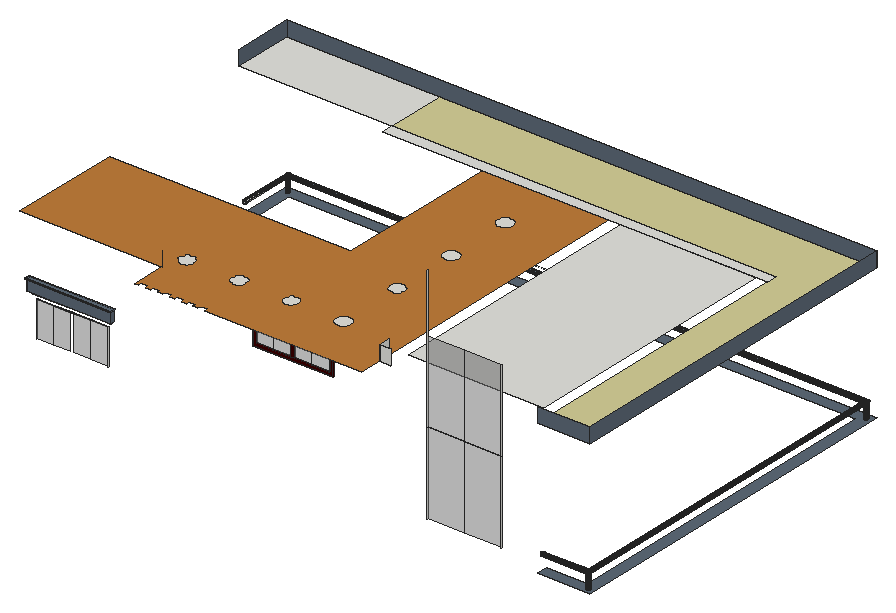
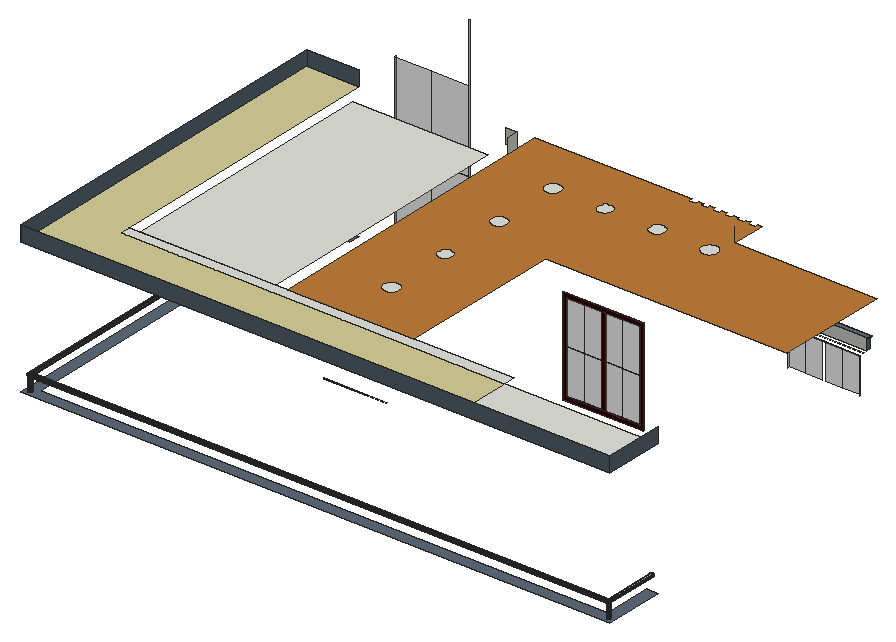
# SketchUp Ruby script. Lengths in inches.
U = 1.inch
M = Sketchup.active_model
def pt(a) = Geom::Point3d.new(a.map { |v| v * U })
def face(e, loops, mat)
  f = e.add_face(loops[0].map { |a| pt(a) })
  loops[1..].each { |l| e.add_face(l.map { |a| pt(a) }).erase! }
  f.material = f.back_material = mat if mat
  f
end
# faces: each face lists its corners as indices into pts; further lists are holes
def faces(e, pts, list, mat = nil) = list.each { |f| face(e, (f[0].is_a?(Array) ? f : [f]).map { |l| l.map { |i| pts[i] } }, mat) }
# xy, xz, yz: faces in a plane at the given z, y or x. An outline is a flat list of corners, or four numbers for a rectangle; further outlines are holes
def ring(l) = l.size == 4 ? [[l[0], l[1]], [l[2], l[1]], [l[2], l[3]], [l[0], l[3]]] : l.each_slice(2).to_a
def flat(e, list, mat, &to3) = list.each { |f| face(e, (f[0].is_a?(Array) ? f : [f]).map { |l| ring(l).map { |u, v| to3.(u, v) } }, mat) }
def xy(e, z, list, mat = nil) = flat(e, list, mat) { |x, y| [x, y, z] }
def xz(e, y, list, mat = nil) = flat(e, list, mat) { |x, z| [x, y, z] }
def yz(e, x, list, mat = nil) = flat(e, list, mat) { |y, z| [x, y, z] }
def lines(e, pts, list) = list.each { |a, b| e.add_line(pt(pts[a]), pt(pts[b])) }
# prism: a flat outline (further loops are holes) pulled along v
def prism(e, loops, v, mat = nil)
  f = face(e, loops, mat); d = Geom::Vector3d.new(v.map { |x| x * U })
  f.pushpull(f.normal.samedirection?(d) ? d.length : -d.length)
end
def box(e, o, s, mat = nil) = prism(e, [[o, [o[0] + s[0], o[1], o[2]], [o[0] + s[0], o[1] + s[1], o[2]], [o[0], o[1] + s[1], o[2]]]], [0, 0, s[2]], mat)
def at(x, y, z, deg = 0) = Geom::Transformation.translation(pt([x, y, z])) * Geom::Transformation.rotation(ORIGIN, Z_AXIS, deg.degrees)
def axes(o, x, y, z) = Geom::Transformation.new([*x, 0, *y, 0, *z, 0, *pt(o).to_a, 1])
def part(name) = M.definitions.add(name)
# library, detail: a bought-in or finely detailed component or shape, given as its bounding box
def library(name, o, s) = part(name).tap { |d| box(d.entities, o, s) }
def detail(e, o, s) = box(e.add_group.entities, o, s)
def put(e, d, t, mat = nil) = e.add_instance(d, t).tap { |i| i.material = mat if mat }
def group(e, t, mat = nil) = e.add_group.tap { |g| g.transformation = t; g.material = mat if mat }.entities
root = M.entities
M.materials.add("[0022_Maroon]").color = [61, 0, 0]
M.materials.add("[0040_Peru]").color = [191, 124, 58]
M.materials.add("[0048_PaleGoldenrod]").color = [211, 206, 151]
M.materials.add("[0111_SlateGray]").color = [93, 106, 119]
M.materials.add("[0137_Black]").color = [0, 0, 0]
M.materials.add("[Translucent Glass Gray]").color = [128, 128, 128]
M.materials["[Translucent Glass Gray]"].alpha = 0.5
xy(root,420,[[939,69,939.3125,69.02,939.625,69.07,939.93,69.15,940.22,69.26,940.5,69.4,940.76,69.57,941.01,69.77,941.23,69.99,941.43,70.24,941.6,70.5,941.74,70.78,941.85,71.07,941.93,71.375,941.98,71.6875,942,72,941.98,72.3125,941.93,72.625,941.85,72.93,941.74,73.22,941.6,73.5,941.43,73.76,941.23,74.01,941.01,74.23,940.76,74.43,940.5,74.6,940.22,74.74,939.93,74.85,939.625,74.93,939.3125,74.98,939,75,938.6875,74.98,938.375,74.93,938.07,74.85,937.78,74.74,937.5,74.6,937.24,74.43,936.99,74.23,936.77,74.01,936.57,73.76,936.4,73.5,936.26,73.22,936.15,72.93,936.07,72.625,936.02,72.3125,936,72,936.02,71.6875,936.07,71.375,936.15,71.07,936.26,70.78,936.4,70.5,936.57,70.24,936.77,69.99,936.99,69.77,937.24,69.57,937.5,69.4,937.78,69.26,938.07,69.15,938.375,69.07,938.6875,69.02],[9,627,9.78,627.1,10.5,627.4,11.12,627.88,11.6,628.5,11.9,629.22,12,630,11.9,630.78,11.6,631.5,11.12,632.12,10.5,632.6,9.78,632.9,9,633,8.22,632.9,7.5,632.6,6.88,632.12,6.4,631.5,6.1,630.78,6,630,6.1,629.22,6.4,628.5,6.88,627.88,7.5,627.4,8.22,627.1],[939,627,939.78,627.1,940.5,627.4,941.12,627.88,941.6,628.5,941.9,629.22,942,630,941.9,630.78,941.6,631.5,941.12,632.12,940.5,632.6,939.78,632.9,939,633,938.22,632.9,937.5,632.6,936.88,632.12,936.4,631.5,936.1,630.78,936,630,936.1,629.22,936.4,628.5,936.88,627.88,937.5,627.4,938.22,627.1]])
xy(root,420,[[[864,63,948,63,948,639,0,639,0,543,18,543,18,621,930,621,930,81,864,81],[939,69,938.6875,69.02,938.375,69.07,938.07,69.15,937.78,69.26,937.5,69.4,937.24,69.57,936.99,69.77,936.77,69.99,936.57,70.24,936.4,70.5,936.26,70.78,936.15,71.07,936.07,71.375,936.02,71.6875,936,72,936.02,72.3125,936.07,72.625,936.15,72.93,936.26,73.22,936.4,73.5,936.57,73.76,936.77,74.01,936.99,74.23,937.24,74.43,937.5,74.6,937.78,74.74,938.07,74.85,938.375,74.93,938.6875,74.98,939,75,939.3125,74.98,939.625,74.93,939.93,74.85,940.22,74.74,940.5,74.6,940.76,74.43,941.01,74.23,941.23,74.01,941.43,73.76,941.6,73.5,941.74,73.22,941.85,72.93,941.93,72.625,941.98,72.3125,942,72,941.98,71.6875,941.93,71.375,941.85,71.07,941.74,70.78,941.6,70.5,941.43,70.24,941.23,69.99,941.01,69.77,940.76,69.57,940.5,69.4,940.22,69.26,939.93,69.15,939.625,69.07,939.3125,69.02],[939,627,938.22,627.1,937.5,627.4,936.88,627.88,936.4,628.5,936.1,629.22,936,630,936.1,630.78,936.4,631.5,936.88,632.12,937.5,632.6,938.22,632.9,939,633,939.78,632.9,940.5,632.6,941.12,632.12,941.6,631.5,941.9,630.78,942,630,941.9,629.22,941.6,628.5,941.12,627.88,940.5,627.4,939.78,627.1],[9,627,8.22,627.1,7.5,627.4,6.88,627.88,6.4,628.5,6.1,629.22,6,630,6.1,630.78,6.4,631.5,6.88,632.12,7.5,632.6,8.22,632.9,9,633,9.78,632.9,10.5,632.6,11.12,632.12,11.6,631.5,11.9,630.78,12,630,11.9,629.22,11.6,628.5,11.12,627.88,10.5,627.4,9.78,627.1]]],"[0111_SlateGray]")
xy(root,441,[[939,69,938.6875,69.02,938.375,69.07,938.07,69.15,937.78,69.26,937.5,69.4,937.24,69.57,936.99,69.77,936.77,69.99,936.57,70.24,936.4,70.5,936.26,70.78,936.15,71.07,936.07,71.375,936.02,71.6875,936,72,939,72,939,75,939.3125,74.98,939.625,74.93,939.93,74.85,940.22,74.74,940.5,74.6,940.76,74.43,941.01,74.23,941.23,74.01,941.43,73.76,941.6,73.5,941.74,73.22,941.85,72.93,941.93,72.625,941.98,72.3125,942,72,941.98,71.6875,941.93,71.375,941.85,71.07,941.74,70.78,941.6,70.5,941.43,70.24,941.23,69.99,941.01,69.77,940.76,69.57,940.5,69.4,940.22,69.26,939.93,69.15,939.625,69.07,939.3125,69.02],[936,72,936.02,72.3125,936.07,72.625,936.15,72.93,936.26,73.22,936.4,73.5,936.57,73.76,936.77,74.01,936.99,74.23,937.24,74.43,937.5,74.6,937.78,74.74,938.07,74.85,938.375,74.93,938.6875,74.98,939,75,939,72],[9,627,8.22,627.1,7.5,627.4,6.88,627.88,6.4,628.5,6.1,629.22,6,630,6.1,630.78,6.4,631.5,6.88,632.12,7.5,632.6,8.22,632.9,9,633,9.78,632.9,10.5,632.6,11.12,632.12,11.6,631.5,11.9,630.78,12,630,9,630],[9,627,9,630,12,630,11.9,629.22,11.6,628.5,11.12,627.88,10.5,627.4,9.78,627.1],[939,627,938.22,627.1,937.5,627.4,936.88,627.88,936.4,628.5,936.1,629.22,936,630,939,630],
  [939,627,939,630,936,630,936.1,630.78,936.4,631.5,936.88,632.12,937.5,632.6,938.22,632.9,939,633,939.78,632.9,940.5,632.6,941.12,632.12,941.6,631.5,941.9,630.78,942,630,941.9,629.22,941.6,628.5,941.12,627.88,940.5,627.4,939.78,627.1]])
xy(root,443.89,[[247.48,261,376.91,262]],"[0022_Maroon]")
xy(root,449.89,[[253.48,261,281.33,262],[281.33,261,309.19,262],[309.19,261,315.19,262],[315.19,261,343.05,262],[343.05,261,370.91,262]])
xy(root,529.0625,[[450.63,525,550.69,526]])
xy(root,531.8125,[[58.65,63,86.31,64],[86.31,63,113.97,64],[113.97,63,117.97,64],[117.97,63,145.62,64],[145.62,63,173.28,64]])
xy(root,537.8125,[[52.65,63,179.28,64]],"[0137_Black]")
xy(root,541.86,[[48.05,57,182.67,63]],"[0111_SlateGray]")
xy(root,559.67,[[46.05,55,46.05,63,48.05,63,48.05,57,182.67,57,182.67,63,184.17,63,184.17,55]],"[0111_SlateGray]")
xy(root,561.17,[[46.05,55,184.17,63]],"[0111_SlateGray]")
xy(root,592.64,[[253.48,261,281.33,262],[281.33,261,309.19,262],[309.19,261,315.19,262],[315.19,261,343.05,262],[343.05,261,370.91,262]])
xy(root,598.64,[[247.48,261,376.91,262]],"[0022_Maroon]")
xy(root,636,[[627.8125,99,846,525],[259.1875,102.45,256.08,102.86,253.1875,104.06,250.7,105.97,248.8,108.45,247.6,111.35,247.1875,114.45,247.6,117.56,248.8,120.45,250.7,122.9375,253.1875,124.84,256.08,126.04,259.1875,126.45,262.29,126.04,265.1875,124.84,267.67,122.9375,269.58,120.45,270.78,117.56,271.1875,114.45,270.78,111.35,269.58,108.45,267.67,105.97,265.1875,104.06,262.29,102.86],[343.1875,102.45,340.08,102.86,337.1875,104.06,334.7,105.97,332.8,108.45,331.6,111.35,331.1875,114.45,331.6,117.56,332.8,120.45,334.7,122.9375,337.1875,124.84,340.08,126.04,343.1875,126.45,346.29,126.04,349.1875,124.84,351.67,122.9375,353.58,120.45,354.78,117.56,355.1875,114.45,354.78,111.35,353.58,108.45,351.67,105.97,349.1875,104.06,346.29,102.86],[427.1875,102.45,424.08,102.86,421.1875,104.06,418.7,105.97,416.8,108.45,415.6,111.35,415.1875,114.45,415.6,117.56,416.8,120.45,418.7,122.9375,421.1875,124.84,424.08,126.04,427.1875,126.45,430.29,126.04,433.1875,124.84,435.67,122.9375,437.58,120.45,438.78,117.56,439.1875,114.45,438.78,111.35,437.58,108.45,435.67,105.97,433.1875,104.06,430.29,102.86],[511.1875,102.45,508.08,102.86,505.1875,104.06,502.7,105.97,500.8,108.45,499.6,111.35,499.1875,114.45,499.6,117.56,500.8,120.45,502.7,122.9375,505.1875,124.84,508.08,126.04,511.1875,126.45,514.29,126.04,517.1875,124.84,519.67,122.9375,521.58,120.45,522.78,117.56,523.1875,114.45,522.78,111.35,521.58,108.45,519.67,105.97,517.1875,104.06,514.29,102.86],
  [511.1875,210.45,508.08,210.86,505.1875,212.06,502.7,213.97,500.8,216.45,499.6,219.35,499.1875,222.45,499.6,225.56,500.8,228.45,502.7,230.9375,505.1875,232.84,508.08,234.04,511.1875,234.45,514.29,234.04,517.1875,232.84,519.67,230.9375,521.58,228.45,522.78,225.56,523.1875,222.45,522.78,219.35,521.58,216.45,519.67,213.97,517.1875,212.06,514.29,210.86],[511.1875,318.45,508.08,318.86,505.1875,320.06,502.7,321.97,500.8,324.45,499.6,327.35,499.1875,330.45,499.6,333.56,500.8,336.45,502.7,338.9375,505.1875,340.84,508.08,342.04,511.1875,342.45,514.29,342.04,517.1875,340.84,519.67,338.9375,521.58,336.45,522.78,333.56,523.1875,330.45,522.78,327.35,521.58,324.45,519.67,321.97,517.1875,320.06,514.29,318.86],[511.1875,426.45,508.08,426.86,505.1875,428.06,502.7,429.97,500.8,432.45,499.6,435.35,499.1875,438.45,499.6,441.56,500.8,444.45,502.7,446.9375,505.1875,448.84,508.08,450.04,511.1875,450.45,514.29,450.04,517.1875,448.84,519.67,446.9375,521.58,444.45,522.78,441.56,523.1875,438.45,522.78,435.35,521.58,432.45,519.67,429.97,517.1875,428.06,514.29,426.86],[246,525,864,543],[0,543,246,639]])
xy(root,636,[[[246,27,246,81,18,81,18,261,405.8125,261,405.8125,525,609.8125,525,609.8125,27,358.5625,27,358.5625,31.875,347.375,31.875,347.375,27,339.36,27,339.36,31.875,328.18,31.875,328.18,27,320.16,27,320.16,31.875,308.98,31.875,308.98,27,300.96,27,300.96,31.875,289.78,31.875,289.78,27,281.76,27,281.76,31.875,270.58,31.875,270.58,27,262.5625,27,262.5625,31.875,251.375,31.875,251.375,27],[511.1875,426.45,514.29,426.86,517.1875,428.06,519.67,429.97,521.58,432.45,522.78,435.35,523.1875,438.45,522.78,441.56,521.58,444.45,519.67,446.9375,517.1875,448.84,514.29,450.04,511.1875,450.45,508.08,450.04,505.1875,448.84,502.7,446.9375,500.8,444.45,499.6,441.56,499.1875,438.45,499.6,435.35,500.8,432.45,502.7,429.97,505.1875,428.06,508.08,426.86],[511.1875,318.45,514.29,318.86,517.1875,320.06,519.67,321.97,521.58,324.45,522.78,327.35,523.1875,330.45,522.78,333.56,521.58,336.45,519.67,338.9375,517.1875,340.84,514.29,342.04,511.1875,342.45,508.08,342.04,505.1875,340.84,502.7,338.9375,500.8,336.45,499.6,333.56,499.1875,330.45,499.6,327.35,500.8,324.45,502.7,321.97,505.1875,320.06,508.08,318.86],[511.1875,210.45,514.29,210.86,517.1875,212.06,519.67,213.97,521.58,216.45,522.78,219.35,523.1875,222.45,522.78,225.56,521.58,228.45,519.67,230.9375,517.1875,232.84,514.29,234.04,511.1875,234.45,508.08,234.04,505.1875,232.84,502.7,230.9375,500.8,228.45,499.6,225.56,499.1875,222.45,499.6,219.35,500.8,216.45,502.7,213.97,505.1875,212.06,508.08,210.86],[511.1875,102.45,514.29,102.86,517.1875,104.06,519.67,105.97,521.58,108.45,522.78,111.35,523.1875,114.45,522.78,117.56,521.58,120.45,519.67,122.9375,517.1875,124.84,514.29,126.04,511.1875,126.45,508.08,126.04,505.1875,124.84,502.7,122.9375,500.8,120.45,499.6,117.56,499.1875,114.45,499.6,111.35,500.8,108.45,502.7,105.97,505.1875,104.06,508.08,102.86],[427.1875,102.45,430.29,102.86,433.1875,104.06,435.67,105.97,437.58,108.45,438.78,111.35,439.1875,114.45,438.78,117.56,437.58,120.45,435.67,122.9375,433.1875,124.84,430.29,126.04,427.1875,126.45,424.08,126.04,421.1875,124.84,418.7,122.9375,416.8,120.45,415.6,117.56,415.1875,114.45,415.6,111.35,416.8,108.45,418.7,105.97,421.1875,104.06,424.08,102.86],[343.1875,102.45,346.29,102.86,349.1875,104.06,351.67,105.97,353.58,108.45,354.78,111.35,355.1875,114.45,354.78,117.56,353.58,120.45,351.67,122.9375,349.1875,124.84,346.29,126.04,343.1875,126.45,340.08,126.04,337.1875,124.84,334.7,122.9375,332.8,120.45,331.6,117.56,331.1875,114.45,331.6,111.35,332.8,108.45,334.7,105.97,337.1875,104.06,340.08,102.86],[259.1875,102.45,262.29,102.86,265.1875,104.06,267.67,105.97,269.58,108.45,270.78,111.35,271.1875,114.45,270.78,117.56,269.58,120.45,267.67,122.9375,265.1875,124.84,262.29,126.04,259.1875,126.45,256.08,126.04,253.1875,124.84,250.7,122.9375,248.8,120.45,247.6,117.56,247.1875,114.45,247.6,111.35,248.8,108.45,250.7,105.97,253.1875,104.06,256.08,102.86]]],"[0040_Peru]")
xy(root,636,[[864,63,864,543,246,543,246,639,948,639,948,63]],"[0048_PaleGoldenrod]")
xz(root,55,[[46.05,559.67,184.17,561.17]],"[0111_SlateGray]")
xz(root,57,[[48.05,541.86,182.67,559.67]],"[0111_SlateGray]")
xz(root,63,[[48.05,541.86,182.67,561.17],[46.05,559.67,48.05,561.17],[182.67,559.67,184.17,561.17],[609.8125,636,627.8125,660]])
xz(root,63,[[864,636,948,660]],"[0111_SlateGray]")
xz(root,63,[[687,435.72,746.59,567.72],[746.59,435.72,806.18,567.72],[58.65,474.5,86.31,531.8125],[86.31,474.5,113.97,531.8125],[117.97,474.5,145.62,531.8125],
  [145.62,474.5,173.28,531.8125],[687,567.72,746.59,699.72],[746.59,567.72,806.18,699.72]],"[Translucent Glass Gray]")
xz(root,261,[[309.19,449.89,315.19,592.64]],"[0022_Maroon]")
xz(root,261,[[253.48,449.89,281.33,521.26],[281.33,449.89,309.19,521.26],[315.19,449.89,343.05,521.26],[343.05,449.89,370.91,521.26],[253.48,521.26,281.33,592.64],
  [281.33,521.26,309.19,592.64],[315.19,521.26,343.05,592.64],[343.05,521.26,370.91,592.64]],"[Translucent Glass Gray]")
xz(root,262,[[[247.48,443.89,376.91,598.64],[253.48,449.89,370.91,592.64]]],"[0022_Maroon]")
xz(root,543,[[9,441,9.78,441.1,10.5,441.4,11.12,441.88,11.6,442.5,11.9,443.22,12,444,11.9,444.78,11.6,445.5,11.12,446.12,10.5,446.6,9.78,446.9,9,447,8.22,446.9,7.5,446.6,6.88,446.12,6.4,445.5,6.1,444.78,6,444,6.1,443.22,6.4,442.5,6.88,441.88,7.5,441.4,8.22,441.1]])
xz(root,639,[[0,636,948,660]],"[0111_SlateGray]")
yz(root,0,[[543,636,639,660]],"[0111_SlateGray]")
yz(root,46.05,[[55,559.67,57,561.17],[57,559.67,63,561.17]],"[0111_SlateGray]")
yz(root,48.05,[[57,541.86,63,559.67]],"[0111_SlateGray]")
yz(root,58.65,[[63,474.5,64,531.8125]])
yz(root,173.28,[[63,474.5,64,531.8125]])
yz(root,182.67,[[57,541.86,63,559.67]],"[0111_SlateGray]")
yz(root,184.17,[[55,559.67,63,561.17]],"[0111_SlateGray]")
yz(root,247.48,[[261,443.89,262,598.64]],"[0022_Maroon]")
yz(root,253.48,[[261,449.89,262,521.26],[261,521.26,262,592.64]])
yz(root,370.91,[[261,449.89,262,521.26],[261,521.26,262,592.64]])
yz(root,376.91,[[261,443.89,262,598.64]],"[0022_Maroon]")
yz(root,609.8125,[[63,636,81,660]])
yz(root,687,[[62,435.72,63,567.72],[62,567.72,63,793.97]])
yz(root,806.18,[[62,435.72,63,567.72],[62,567.72,63,699.72]])
yz(root,948,[[63,636,639,660]],"[0111_SlateGray]")
p = [[938.6875,69.02,420],[938.375,69.07,420],[938.375,69.07,441],[938.6875,69.02,441],[939,69,420],[939,69,441],
  [939.3125,69.02,420],[939.3125,69.02,441],[939.625,69.07,420],[939.625,69.07,441],[938.07,69.15,420],[937.78,69.26,420],
  [937.78,69.26,441],[938.07,69.15,441],[939.93,69.15,420],[939.93,69.15,441],[940.22,69.26,420],[940.22,69.26,441],
  [937.5,69.4,420],[937.5,69.4,441],[940.5,69.4,420],[940.5,69.4,441],[937.24,69.57,420],[937.24,69.57,441],
  [940.76,69.57,420],[940.76,69.57,441],[936.99,69.77,420],[936.99,69.77,441],[941.01,69.77,420],[941.01,69.77,441],
  [936.77,69.99,420],[936.77,69.99,441],[941.23,69.99,420],[941.23,69.99,441],[936.57,70.24,420],[936.57,70.24,441],
  [941.43,70.24,420],[941.43,70.24,441],[936.4,70.5,420],[936.4,70.5,441],[941.6,70.5,420],[941.6,70.5,441],
  [936.26,70.78,420],[936.26,70.78,441],[941.74,70.78,420],[941.74,70.78,441],[936.15,71.07,420],[936.15,71.07,441],
  [941.85,71.07,420],[941.85,71.07,441],[936.07,71.375,420],[936.07,71.375,441],[941.93,71.375,420],[941.93,71.375,441],
  [936.02,71.6875,420],[936.02,71.6875,441],[941.98,71.6875,420],[941.98,71.6875,441],[936,72,420],[936,72,441],
  [942,72,420],[942,72,441],[936.02,72.3125,420],[936.02,72.3125,441],[941.98,72.3125,420],[941.98,72.3125,441],
  [936.07,72.625,420],[936.07,72.625,441],[941.93,72.625,420],[941.93,72.625,441],[936.15,72.93,420],[936.15,72.93,441],
  [941.85,72.93,420],[941.85,72.93,441],[936.26,73.22,420],[936.26,73.22,441],[941.74,73.22,420],[941.74,73.22,441],
  [936.4,73.5,420],[936.4,73.5,441],[941.6,73.5,420],[941.6,73.5,441],[936.57,73.76,420],[936.57,73.76,441],
  [941.43,73.76,420],[941.43,73.76,441],[936.77,74.01,420],[936.77,74.01,441],[941.23,74.01,420],[941.23,74.01,441],
  [936.99,74.23,420],[936.99,74.23,441],[941.01,74.23,420],[941.01,74.23,441],[937.24,74.43,420],[937.24,74.43,441],
  [940.76,74.43,420],[940.76,74.43,441],[937.5,74.6,420],[937.5,74.6,441],[940.5,74.6,420],[940.5,74.6,441],
  [937.78,74.74,420],[937.78,74.74,441],[940.22,74.74,420],[940.22,74.74,441],[938.07,74.85,420],[938.07,74.85,441],
  [939.93,74.85,420],[939.93,74.85,441],[938.375,74.93,420],[938.375,74.93,441],[938.6875,74.98,420],[938.6875,74.98,441],
  [939.3125,74.98,420],[939.625,74.93,420],[939.625,74.93,441],[939.3125,74.98,441],[939,75,420],[939,75,441],
  [9,627,420],[8.22,627.1,420],[8.22,627.1,441],[9,627,441],[9.78,627.1,420],[9.78,627.1,441],
  [939,627,420],[938.22,627.1,420],[938.22,627.1,441],[939,627,441],[939.78,627.1,420],[939.78,627.1,441],
  [7.5,627.4,420],[7.5,627.4,441],[10.5,627.4,420],[10.5,627.4,441],[937.5,627.4,420],[937.5,627.4,441],
  [940.5,627.4,420],[940.5,627.4,441],[6.88,627.88,420],[6.88,627.88,441],[11.12,627.88,420],[11.12,627.88,441],
  [936.88,627.88,420],[936.88,627.88,441],[941.12,627.88,420],[941.12,627.88,441],[6.4,628.5,420],[6.4,628.5,441],
  [11.6,628.5,420],[11.6,628.5,441],[936.4,628.5,420],[936.4,628.5,441],[941.6,628.5,420],[941.6,628.5,441],
  [6.1,629.22,420],[6.1,629.22,441],[11.9,629.22,420],[11.9,629.22,441],[936.1,629.22,420],[936.1,629.22,441],
  [941.9,629.22,420],[941.9,629.22,441],[6,630,420],[6,630,441],[12,630,420],[12,630,441],
  [936,630,420],[936,630,441],[942,630,420],[942,630,441],[6.1,630.78,420],[6.1,630.78,441],
  [11.9,630.78,420],[11.9,630.78,441],[936.1,630.78,420],[936.1,630.78,441],[941.9,630.78,420],[941.9,630.78,441],
  [6.4,631.5,420],[6.4,631.5,441],[11.6,631.5,420],[11.6,631.5,441],[936.4,631.5,420],[936.4,631.5,441],
  [941.6,631.5,420],[941.6,631.5,441],[6.88,632.12,420],[6.88,632.12,441],[11.12,632.12,420],[11.12,632.12,441],
  [936.88,632.12,420],[936.88,632.12,441],[941.12,632.12,420],[941.12,632.12,441],[7.5,632.6,420],[7.5,632.6,441],
  [10.5,632.6,420],[10.5,632.6,441],[937.5,632.6,420],[937.5,632.6,441],[940.5,632.6,420],[940.5,632.6,441],
  [8.22,632.9,420],[8.22,632.9,441],[9.78,632.9,420],[9.78,632.9,441],[938.22,632.9,420],[938.22,632.9,441],
  [939.78,632.9,420],[939.78,632.9,441],[9,633,420],[9,633,441],[939,633,420],[939,633,441],
  [939,72,441],[939.78,71.22,441.1],[864,71.22,441.1],[864,72,441],[939,630,441],[939.78,630.78,441.1],
  [938.22,72.78,441.1],[864,72.78,441.1],[938.22,629.22,441.1],[9,543,441],[8.22,543,441.1],[8.22,630.78,441.1],
  [9,630,441],[9.78,543,441.1],[9.78,629.22,441.1],[940.5,70.5,441.4],[864,70.5,441.4],[940.5,631.5,441.4],
  [937.5,73.5,441.4],[864,73.5,441.4],[937.5,628.5,441.4],[7.5,543,441.4],[7.5,631.5,441.4],[10.5,543,441.4],
  [10.5,628.5,441.4],[941.12,69.88,441.88],[864,69.88,441.88],[941.12,632.12,441.88],[936.88,74.12,441.88],[864,74.12,441.88],
  [936.88,627.88,441.88],[6.88,543,441.88],[6.88,632.12,441.88],[11.12,543,441.88],[11.12,627.88,441.88],[941.6,69.4,442.5],
  [864,69.4,442.5],[941.6,632.6,442.5],[936.4,74.6,442.5],[864,74.6,442.5],[936.4,627.4,442.5],[6.4,543,442.5],
  [6.4,632.6,442.5],[11.6,543,442.5],[11.6,627.4,442.5],[941.9,69.1,443.22],[864,69.1,443.22],[941.9,632.9,443.22],
  [936.1,74.9,443.22],[864,74.9,443.22],[936.1,627.1,443.22],[6.1,543,443.22],[6.1,632.9,443.22],[11.9,543,443.22],
  [11.9,627.1,443.22],[942,69,444],[864,69,444],[942,633,444],[936,75,444],[864,75,444],
  [936,627,444],[6,543,444],[6,633,444],[12,543,444],[12,627,444],[941.9,69.1,444.78],
  [864,69.1,444.78],[941.9,632.9,444.78],[936.1,74.9,444.78],[864,74.9,444.78],[936.1,627.1,444.78],[6.1,543,444.78],
  [6.1,632.9,444.78],[11.9,543,444.78],[11.9,627.1,444.78],[941.6,69.4,445.5],[864,69.4,445.5],[941.6,632.6,445.5],
  [936.4,74.6,445.5],[864,74.6,445.5],[936.4,627.4,445.5],[6.4,543,445.5],[6.4,632.6,445.5],[11.6,543,445.5],
  [11.6,627.4,445.5],[941.12,69.88,446.12],[864,69.88,446.12],[941.12,632.12,446.12],[936.88,74.12,446.12],[864,74.12,446.12],
  [936.88,627.88,446.12],[6.88,543,446.12],[6.88,632.12,446.12],[11.12,543,446.12],[11.12,627.88,446.12],[940.5,70.5,446.6],
  [864,70.5,446.6],[940.5,631.5,446.6],[937.5,73.5,446.6],[864,73.5,446.6],[937.5,628.5,446.6],[7.5,543,446.6],
  [7.5,631.5,446.6],[10.5,543,446.6],[10.5,628.5,446.6],[939.78,71.22,446.9],[864,71.22,446.9],[939.78,630.78,446.9],
  [938.22,72.78,446.9],[864,72.78,446.9],[938.22,629.22,446.9],[8.22,543,446.9],[8.22,630.78,446.9],[9.78,543,446.9],
  [9.78,629.22,446.9],[939,72,447],[864,72,447],[939,630,447],[9,543,447],[9,630,447],
  [48.05,57,559.67],[48.05,57,561.17],[246,81,636],[246,81,660],[939,72,420],[939,72,444],
  [864,72,444],[939,630,420],[939,630,444],[9,630,420],[9,630,444],[9,543,444]]
faces(root,p,[[0,1,2,3],[4,0,3,5],[6,4,5,7],[8,6,7,9],[10,11,12,13],[1,10,13,2],[14,8,9,15],[16,14,15,17],
  [11,18,19,12],[20,16,17,21],[18,22,23,19],[24,20,21,25],[22,26,27,23],[28,24,25,29],[26,30,31,27],[32,28,29,33],
  [30,34,35,31],[36,32,33,37],[34,38,39,35],[40,36,37,41],[38,42,43,39],[44,40,41,45],[42,46,47,43],[48,44,45,49],
  [46,50,51,47],[52,48,49,53],[50,54,55,51],[56,52,53,57],[54,58,59,55],[60,56,57,61],[58,62,63,59],[64,60,61,65],
  [62,66,67,63],[68,64,65,69],[66,70,71,67],[72,68,69,73],[70,74,75,71],[76,72,73,77],[74,78,79,75],[80,76,77,81],
  [78,82,83,79],[84,80,81,85],[82,86,87,83],[88,84,85,89],[86,90,91,87],[92,88,89,93],[90,94,95,91],[96,92,93,97],
  [94,98,99,95],[100,96,97,101],[98,102,103,99],[104,100,101,105],[102,106,107,103],[108,104,105,109],[106,110,111,107],[110,112,113,111],
  [114,115,116,117],[115,108,109,116],[112,118,119,113],[118,114,117,119],[126,127,128,129],[130,126,129,131],[127,136,137,128],[138,130,131,139],
  [136,144,145,137],[146,138,139,147],[144,152,153,145],[154,146,147,155],[152,160,161,153],[162,154,155,163],[160,168,169,161],[170,162,163,171],
  [168,176,177,169],[178,170,171,179],[176,184,185,177],[186,178,179,187],[184,192,193,185],[194,186,187,195],[192,200,201,193],[202,194,195,203],
  [200,208,209,201],[210,202,203,211],[208,214,215,209],[214,210,211,215],[216,217,218,219,59],[220,221,217,216,119,129],[222,216,59,219,223],[224,220,129,119,216,222],
  [230,228,167,169,220,224],[228,227,221,220,169,167],[217,231,232,218],[221,233,231,217],[234,222,223,235],[236,224,222,234],[240,230,224,236],[227,238,233,221],
  [231,241,242,232],[233,243,241,231],[244,234,235,245],[246,236,234,244],[250,240,236,246],[238,248,243,233],[241,251,252,242],[243,253,251,241],
  [254,244,245,255],[256,246,244,254],[260,250,246,256],[248,258,253,243],[251,261,262,252],[253,263,261,251],[264,254,255,265],[266,256,254,264],
  [270,260,256,266],[258,268,263,253],[261,271,272,262],[263,273,271,261],[274,264,265,275],[276,266,264,274],[280,270,266,276],[268,278,273,263],
  [271,281,282,272],[273,283,281,271],[284,274,275,285],[286,276,274,284],[290,280,276,286],[278,288,283,273],[281,291,292,282],[283,293,291,281],
  [294,284,285,295],[296,286,284,294],[300,290,286,296],[288,298,293,283],[291,301,302,292],[293,303,301,291],[304,294,295,305],[306,296,294,304],
  [310,300,296,306],[298,308,303,293],[301,311,312,302],[303,313,311,301],[314,304,305,315],[316,306,304,314],[320,310,306,316],[308,318,313,303],
  [311,321,322,312],[313,323,321,311],[324,314,315,325],[326,316,314,324],[330,320,316,326],[318,328,323,313],[321,331,332,322],[323,333,331,321],
  [331,324,325,332],[333,326,324,331],[335,330,326,333],[328,335,333,323]],"[0111_SlateGray]")
faces(root,p,[[120,121,122,123],[124,120,123,125],[121,132,133,122],[134,124,125,135],[132,140,141,133],[142,134,135,143],[140,148,149,141],[150,142,143,151],
  [148,156,157,149],[158,150,151,159],[156,164,165,157],[166,158,159,167],[164,172,173,165],[174,166,167,175],[172,180,181,173],[182,174,175,183],
  [180,188,189,181],[190,182,183,191],[188,196,197,189],[198,190,191,199],[196,204,205,197],[206,198,199,207],[204,212,213,205],[212,206,207,213],
  [225,226,227,228,123],[229,225,123,228,230],[226,237,238,227],[239,229,230,240],[237,247,248,238],[249,239,240,250],[247,257,258,248],[259,249,250,260],
  [257,267,268,258],[269,259,260,270],[267,277,278,268],[279,269,270,280],[277,287,288,278],[289,279,280,290],[287,297,298,288],[299,289,290,300],
  [297,307,308,298],[309,299,300,310],[307,317,318,308],[319,309,310,320],[317,327,328,318],[329,319,320,330],[327,334,335,328],[334,329,330,335]])
lines(root,p,[[336,337],[338,339],[340,216],[341,342],[343,220],[344,341],[345,228],[346,344],[346,347],[216,341],[220,344],[228,346]])
